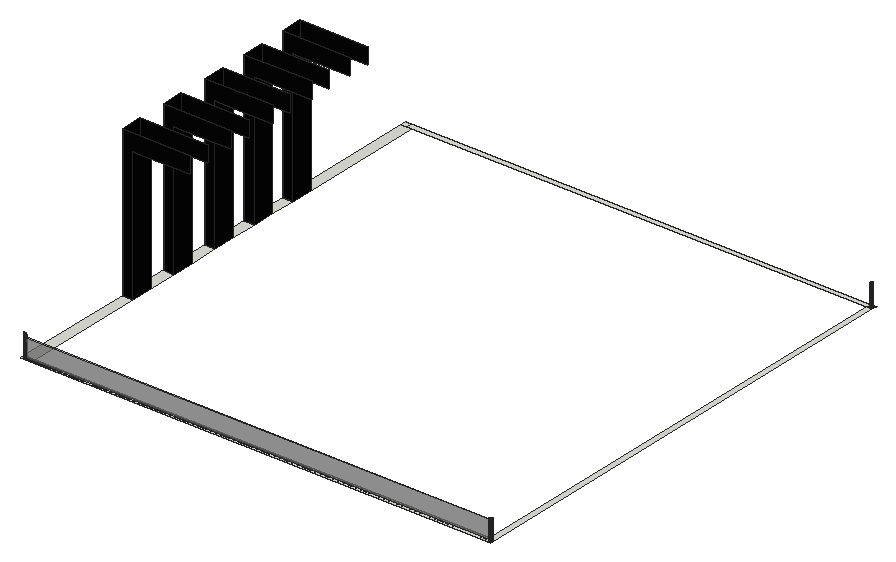
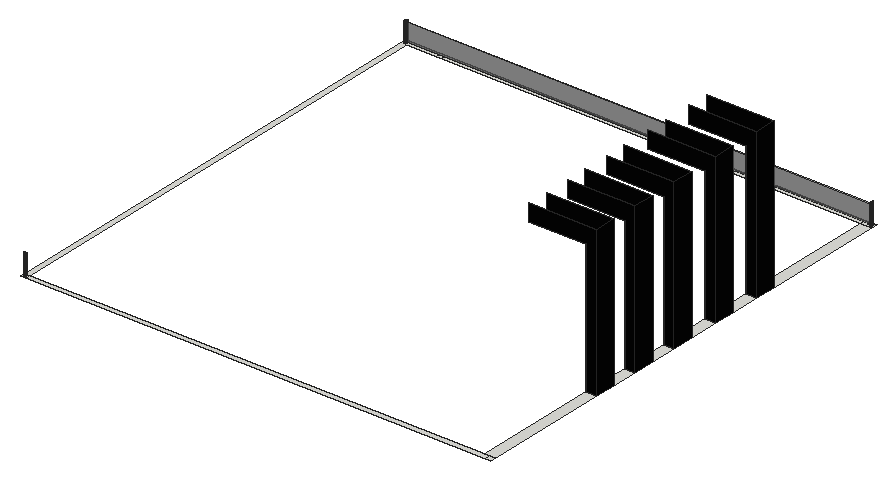
# SketchUp Ruby script. Lengths in inches.
U = 1.inch
M = Sketchup.active_model
def pt(a) = Geom::Point3d.new(a.map { |v| v * U })
def face(e, loops, mat)
  f = e.add_face(loops[0].map { |a| pt(a) })
  loops[1..].each { |l| e.add_face(l.map { |a| pt(a) }).erase! }
  f.material = f.back_material = mat if mat
  f
end
# faces: each face lists its corners as indices into pts; further lists are holes
def faces(e, pts, list, mat = nil) = list.each { |f| face(e, (f[0].is_a?(Array) ? f : [f]).map { |l| l.map { |i| pts[i] } }, mat) }
# xy, xz, yz: faces in a plane at the given z, y or x. An outline is a flat list of corners, or four numbers for a rectangle; further outlines are holes
def ring(l) = l.size == 4 ? [[l[0], l[1]], [l[2], l[1]], [l[2], l[3]], [l[0], l[3]]] : l.each_slice(2).to_a
def flat(e, list, mat, &to3) = list.each { |f| face(e, (f[0].is_a?(Array) ? f : [f]).map { |l| ring(l).map { |u, v| to3.(u, v) } }, mat) }
def xy(e, z, list, mat = nil) = flat(e, list, mat) { |x, y| [x, y, z] }
def xz(e, y, list, mat = nil) = flat(e, list, mat) { |x, z| [x, y, z] }
def yz(e, x, list, mat = nil) = flat(e, list, mat) { |y, z| [x, y, z] }
def lines(e, pts, list) = list.each { |a, b| e.add_line(pt(pts[a]), pt(pts[b])) }
# prism: a flat outline (further loops are holes) pulled along v
def prism(e, loops, v, mat = nil)
  f = face(e, loops, mat); d = Geom::Vector3d.new(v.map { |x| x * U })
  f.pushpull(f.normal.samedirection?(d) ? d.length : -d.length)
end
def box(e, o, s, mat = nil) = prism(e, [[o, [o[0] + s[0], o[1], o[2]], [o[0] + s[0], o[1] + s[1], o[2]], [o[0], o[1] + s[1], o[2]]]], [0, 0, s[2]], mat)
def at(x, y, z, deg = 0) = Geom::Transformation.translation(pt([x, y, z])) * Geom::Transformation.rotation(ORIGIN, Z_AXIS, deg.degrees)
def axes(o, x, y, z) = Geom::Transformation.new([*x, 0, *y, 0, *z, 0, *pt(o).to_a, 1])
def part(name) = M.definitions.add(name)
# library, detail: a bought-in or finely detailed component or shape, given as its bounding box
def library(name, o, s) = part(name).tap { |d| box(d.entities, o, s) }
def detail(e, o, s) = box(e.add_group.entities, o, s)
def put(e, d, t, mat = nil) = e.add_instance(d, t).tap { |i| i.material = mat if mat }
def group(e, t, mat = nil) = e.add_group.tap { |g| g.transformation = t; g.material = mat if mat }.entities
root = M.entities
M.materials.add("[0136_Charcoal]").color = [5, 5, 5]
M.materials.add("[0137_Black]").color = [0, 0, 0]
M.materials.add("[Translucent Glass Gray]").color = [128, 128, 128]
M.materials["[Translucent Glass Gray]"].alpha = 0.5
xy(root,1309.0625,[[0,72.375,12,72.375,12,75.58,8.99,75.58,8.99,78.17,8.98,78.0625,8.93,77.75,8.85,77.45,8.74,77.15,8.6,76.875,8.43,76.61,8.23,76.37,8.01,76.15,7.76,75.95,7.5,75.78,7.22,75.63,6.93,75.52,6.625,75.44,6.3125,75.39,6,75.375,5.6875,75.39,5.375,75.44,5.07,75.52,4.78,75.63,4.5,75.78,4.24,75.95,3.99,76.15,3.77,76.37,3.57,76.61,3.4,76.875,3.26,77.15,3.15,77.45,3.07,77.75,3.02,78.0625,3,78.375,3.02,78.6875,3.07,79,3.15,79.3,3.26,79.6,3.4,79.875,3.57,80.14,3.77,80.38,3.99,80.6,4.24,80.8,4.5,80.97,4.78,81.12,5.07,81.23,5.375,81.31,5.6875,81.36,6,81.375,6.3125,81.36,6.625,81.31,6.93,81.23,7.22,81.12,7.5,80.97,7.76,80.8,8.01,80.6,8.23,80.38,8.43,80.14,8.6,79.875,8.74,79.6,8.85,79.3,8.93,79,8.98,78.6875,8.99,78.58,12,78.58,12,84.375,0,84.375],[12,72.375,1086,72.375,1086,1170.375,1074,1170.375,1074,84.375,12,84.375,12,78.58,1077.01,78.58,1077.04,78.89,1077.11,79.2,1077.22,79.49,1077.35,79.78,1077.51,80.05,1077.7,80.3,1077.91,80.53,1078.15,80.74,1078.41,80.92,1078.68,81.07,1078.97,81.19,1079.27,81.28,1079.58,81.35,1079.89,81.37,1080.2,81.37,1080.52,81.33,1080.82,81.26,1081.12,81.16,1081.4,81.03,1081.67,80.86,1081.92,80.68,1082.15,80.46,1082.36,80.23,1082.54,79.97,1082.69,79.69,1082.82,79.41,1082.91,79.11,1082.97,78.8,1083,78.48,1082.99,78.17,1082.96,77.86,1082.89,77.55,1082.78,77.26,1082.65,76.97,1082.49,76.7,1082.3,76.45,1082.09,76.22,1081.85,76.01,1081.59,75.83,1081.32,75.68,1081.03,75.56,1080.73,75.47,1080.42,75.4,1080.11,75.38,1079.8,75.38,1079.48,75.42,1079.18,75.49,1078.88,75.59,1078.6,75.72,1078.33,75.89,1078.08,76.07,1077.85,76.29,1077.64,76.52,1077.46,76.78,1077.31,77.06,1077.18,77.34,1077.09,77.64,1077.03,77.95,1077.01,78.21,1077.01,75.58,12,75.58],[6,75.375,5.6875,75.39,5.375,75.44,5.07,75.52,4.78,75.63,4.5,75.78,4.24,75.95,3.99,76.15,3.77,76.37,3.57,76.61,3.4,76.875,3.26,77.15,3.15,77.45,3.07,77.75,3.02,78.0625,3,78.375,3.02,78.6875,3.07,79,3.15,79.3,3.26,79.6,3.4,79.875,3.57,80.14,3.77,80.38,3.99,80.6,4.24,80.8,4.5,80.97,4.78,81.12,5.07,81.23,5.375,81.31,5.6875,81.36,6,81.375,6.3125,81.36,6.625,81.31,6.93,81.23,7.22,81.12,7.5,80.97,7.76,80.8,8.01,80.6,8.23,80.38,8.43,80.14,8.6,79.875,8.74,79.6,8.85,79.3,8.93,79,8.98,78.6875,8.99,78.58,8.99,78.17,8.98,78.0625,8.93,77.75,8.85,77.45,8.74,77.15,8.6,76.875,8.43,76.61,8.23,76.37,8.01,76.15,7.76,75.95,7.5,75.78,7.22,75.63,6.93,75.52,6.625,75.44,6.3125,75.39],[1079.8,75.38,1079.48,75.42,1079.18,75.49,1078.88,75.59,1078.6,75.72,1078.33,75.89,1078.08,76.07,1077.85,76.29,1077.64,76.52,1077.46,76.78,1077.31,77.06,1077.18,77.34,1077.09,77.64,1077.03,77.95,1077.01,78.21,1077.01,78.58,1077.04,78.89,1077.11,79.2,1077.22,79.49,1077.35,79.78,1077.51,80.05,1077.7,80.3,1077.91,80.53,1078.15,80.74,1078.41,80.92,1078.68,81.07,1078.97,81.19,1079.27,81.28,1079.58,81.35,1079.89,81.37,1080.2,81.37,1080.52,81.33,1080.82,81.26,1081.12,81.16,1081.4,81.03,1081.67,80.86,1081.92,80.68,1082.15,80.46,1082.36,80.23,1082.54,79.97,1082.69,79.69,1082.82,79.41,1082.91,79.11,1082.97,78.8,1083,78.48,1082.99,78.17,1082.96,77.86,1082.89,77.55,1082.78,77.26,1082.65,76.97,1082.49,76.7,1082.3,76.45,1082.09,76.22,1081.85,76.01,1081.59,75.83,1081.32,75.68,1081.03,75.56,1080.73,75.47,1080.42,75.4,1080.11,75.38],[8.99,75.58,8.99,78.17,9,78.375,8.99,78.58,12,78.58,12,75.58],
  [12,75.58,12,78.58,1077.01,78.58,1077,78.27,1077.01,78.21,1077.01,75.58],[8.99,78.17,8.99,78.58,9,78.375],[1077.01,78.21,1077,78.27,1077.01,78.58],[0,84.375,24.25,366.56],[0,366.56,24.25,417.12],
  [0,417.12,24.25,484.62],[0,484.62,24.25,535.18],[0,535.18,24.25,604.12],[0,604.12,24.25,654.68],[0,654.68,24.25,717.12],
  [0,717.12,24.25,767.68],[0,767.68,24.25,827.68],[0,827.68,24.25,878.24],[0,878.24,24.25,1170.375],[0,1170.375,12,1182.375],
  [12,1170.375,1074,1182.375],[[1074,1170.375,1086,1182.375],[1079.86,1173.38,1079.55,1173.41,1079.24,1173.47,1078.94,1173.57,1078.65,1173.69,1078.38,1173.85,1078.125,1174.03,1077.89,1174.24,1077.68,1174.47,1077.49,1174.73,1077.34,1175,1077.21,1175.28,1077.11,1175.58,1077.04,1175.89,1077.01,1176.2,1077,1176.51,1077.03,1176.83,1077.1,1177.13,1077.19,1177.43,1077.32,1177.72,1077.47,1177.99,1077.66,1178.25,1077.87,1178.48,1078.1,1178.69,1078.35,1178.88,1078.62,1179.04,1078.91,1179.17,1079.21,1179.27,1079.51,1179.34,1079.82,1179.37,1080.14,1179.37,1080.45,1179.34,1080.76,1179.28,1081.06,1179.18,1081.35,1179.06,1081.62,1178.9,1081.875,1178.72,1082.11,1178.51,1082.32,1178.28,1082.51,1178.02,1082.66,1177.75,1082.79,1177.47,1082.89,1177.17,1082.96,1176.86,1082.99,1176.55,1083,1176.24,1082.97,1175.92,1082.9,1175.62,1082.81,1175.32,1082.68,1175.03,1082.53,1174.76,1082.34,1174.5,1082.13,1174.27,1081.9,1174.06,1081.65,1173.87,1081.38,1173.71,1081.09,1173.58,1080.79,1173.48,1080.49,1173.41,1080.18,1173.38]],[1079.86,1173.38,1079.55,1173.41,1079.24,1173.47,1078.94,1173.57,1078.65,1173.69,1078.38,1173.85,1078.125,1174.03,1077.89,1174.24,1077.68,1174.47,1077.49,1174.73,1077.34,1175,1077.21,1175.28,1077.11,1175.58,1077.04,1175.89,1077.01,1176.2,1077,1176.51,1077.03,1176.83,1077.1,1177.13,1077.19,1177.43,1077.32,1177.72,1077.47,1177.99,1077.66,1178.25,1077.87,1178.48,1078.1,1178.69,1078.35,1178.88,1078.62,1179.04,1078.91,1179.17,1079.21,1179.27,1079.51,1179.34,1079.82,1179.37,1080.14,1179.37,1080.45,1179.34,1080.76,1179.28,1081.06,1179.18,1081.35,1179.06,1081.62,1178.9,1081.875,1178.72,1082.11,1178.51,1082.32,1178.28,1082.51,1178.02,1082.66,1177.75,1082.79,1177.47,1082.89,1177.17,1082.96,1176.86,1082.99,1176.55,1083,1176.24,1082.97,1175.92,1082.9,1175.62,1082.81,1175.32,1082.68,1175.03,1082.53,1174.76,1082.34,1174.5,1082.13,1174.27,1081.9,1174.06,1081.65,1173.87,1081.38,1173.71,1081.09,1173.58,1080.79,1173.48,1080.49,1173.41,1080.18,1173.38]])
xz(root,75.38,[[1079.8,1309.0625,1080.11,1354.0625]],"[0137_Black]")
xz(root,75.58,[[8.99,1309.0625,1077.01,1352.375]],"[Translucent Glass Gray]")
xz(root,78.58,[[8.99,1309.0625,1077.01,1352.375]],"[Translucent Glass Gray]")
xz(root,81.37,[[1079.89,1309.0625,1080.2,1354.0625]],"[0137_Black]")
xz(root,366.56,[[0,1309.0625,24.25,1309.0625,24.25,1614.61,156,1614.61,156,1652.92,0,1652.92]],"[0136_Charcoal]")
xz(root,417.12,[[0,1309.0625,0,1652.92,156,1652.92,156,1614.61,24.25,1614.61,24.25,1309.0625]],"[0136_Charcoal]")
xz(root,484.62,[[0,1309.0625,24.25,1309.0625,24.25,1614.61,156,1614.61,156,1652.92,0,1652.92]],"[0136_Charcoal]")
xz(root,535.18,[[0,1309.0625,0,1652.92,156,1652.92,156,1614.61,24.25,1614.61,24.25,1309.0625]],"[0136_Charcoal]")
xz(root,604.12,[[0,1309.0625,24.25,1309.0625,24.25,1614.61,156,1614.61,156,1652.92,0,1652.92]],"[0136_Charcoal]")
xz(root,654.68,[[0,1309.0625,0,1652.92,156,1652.92,156,1614.61,24.25,1614.61,24.25,1309.0625]],"[0136_Charcoal]")
xz(root,717.12,[[0,1309.0625,24.25,1309.0625,24.25,1614.61,156,1614.61,156,1652.92,0,1652.92]],"[0136_Charcoal]")
xz(root,767.68,[[0,1309.0625,0,1652.92,156,1652.92,156,1614.61,24.25,1614.61,24.25,1309.0625]],"[0136_Charcoal]")
xz(root,827.68,[[0,1309.0625,24.25,1309.0625,24.25,1614.61,156,1614.61,156,1652.92,0,1652.92]],"[0136_Charcoal]")
xz(root,878.24,[[0,1309.0625,0,1652.92,156,1652.92,156,1614.61,24.25,1614.61,24.25,1309.0625]],"[0136_Charcoal]")
xz(root,1173.38,[[1079.86,1309.0625,1080.18,1354.07]],"[0137_Black]")
xz(root,1179.37,[[1079.82,1309.0625,1080.14,1360.06]],"[0137_Black]")
yz(root,0,[[366.56,1309.0625,417.12,1652.92],[484.62,1309.0625,535.18,1652.92],[604.12,1309.0625,654.68,1652.92],[717.12,1309.0625,767.68,1652.92],[827.68,1309.0625,878.24,1652.92]],"[0136_Charcoal]")
yz(root,8.99,[[75.58,1309.0625,78.58,1352.375]])
yz(root,24.25,[[366.56,1309.0625,417.12,1614.61],[484.62,1309.0625,535.18,1614.61],[604.12,1309.0625,654.68,1614.61],[717.12,1309.0625,767.68,1614.61],[827.68,1309.0625,878.24,1614.61]],"[0136_Charcoal]")
yz(root,1077.01,[[75.58,1309.0625,78.58,1352.375]])
p = [[5.07,75.52,1309.0625],[5.375,75.44,1309.0625],[5.375,75.44,1357.6875],[5.07,75.52,1357.99],[5.6875,75.39,1309.0625],[5.6875,75.39,1357.375],
  [6,75.375,1309.0625],[6,75.375,1357.0625],[6.3125,75.39,1309.0625],[6.3125,75.39,1356.75],[6.625,75.44,1309.0625],[6.625,75.44,1356.4375],
  [6.93,75.52,1309.0625],[6.93,75.52,1356.14],[1079.18,75.49,1309.0625],[1079.48,75.42,1309.0625],[1079.48,75.42,1354.0625],[1079.18,75.49,1354.0625],
  [1079.8,75.38,1309.0625],[1079.8,75.38,1354.0625],[1080.11,75.38,1309.0625],[1080.42,75.4,1309.0625],[1080.42,75.4,1354.0625],[1080.11,75.38,1354.0625],
  [1080.73,75.47,1309.0625],[1080.73,75.47,1354.0625],[4.78,75.63,1309.0625],[4.78,75.63,1358.28],[7.22,75.63,1309.0625],[7.22,75.63,1355.84],
  [1078.88,75.59,1309.0625],[1078.88,75.59,1354.0625],[1081.03,75.56,1309.0625],[1081.03,75.56,1354.0625],[4.5,75.78,1309.0625],[4.5,75.78,1358.5625],
  [7.5,75.78,1309.0625],[7.5,75.78,1355.5625],[1078.6,75.72,1309.0625],[1078.6,75.72,1354.0625],[1081.32,75.68,1309.0625],[1081.32,75.68,1354.0625],
  [1078.33,75.89,1309.0625],[1078.33,75.89,1354.0625],[1081.59,75.83,1309.0625],[1081.59,75.83,1354.0625],[4.24,75.95,1309.0625],[4.24,75.95,1358.83],
  [7.76,75.95,1309.0625],[7.76,75.95,1355.3],[1081.85,76.01,1309.0625],[1081.85,76.01,1354.0625],[3.99,76.15,1309.0625],[3.99,76.15,1359.07],
  [8.01,76.15,1309.0625],[8.01,76.15,1355.06],[1078.08,76.07,1309.0625],[1078.08,76.07,1354.0625],[1082.09,76.22,1309.0625],[1082.09,76.22,1354.0625],
  [3.77,76.37,1309.0625],[3.77,76.37,1359.29],[8.23,76.37,1309.0625],[8.23,76.37,1354.83],[1077.85,76.29,1309.0625],[1077.85,76.29,1354.0625],
  [1082.3,76.45,1309.0625],[1082.3,76.45,1354.0625],[1077.64,76.52,1309.0625],[1077.64,76.52,1354.0625],[3.57,76.61,1309.0625],[3.57,76.61,1359.49],
  [8.43,76.61,1309.0625],[8.43,76.61,1354.64],[1077.46,76.78,1309.0625],[1077.46,76.78,1354.0625],[1082.49,76.7,1309.0625],[1082.49,76.7,1354.0625],
  [3.4,76.875,1309.0625],[3.4,76.875,1359.66],[8.6,76.875,1309.0625],[8.6,76.875,1354.46],[1082.65,76.97,1309.0625],[1082.65,76.97,1354.0625],
  [1077.31,77.06,1309.0625],[1077.31,77.06,1354.0625],[3.26,77.15,1309.0625],[3.26,77.15,1359.8],[8.74,77.15,1309.0625],[8.74,77.15,1354.32],
  [1082.78,77.26,1309.0625],[1082.78,77.26,1354.0625],[1077.18,77.34,1309.0625],[1077.18,77.34,1354.0625],[3.15,77.45,1309.0625],[3.15,77.45,1359.92],
  [8.85,77.45,1309.0625],[8.85,77.45,1354.21],[1077.09,77.64,1309.0625],[1077.09,77.64,1354.0625],[1082.89,77.55,1309.0625],[1082.89,77.55,1354.0625],
  [3.07,77.75,1309.0625],[3.07,77.75,1360],[8.93,77.75,1309.0625],[8.93,77.75,1354.13],[1077.03,77.95,1309.0625],[1077.03,77.95,1354.0625],
  [1082.96,77.86,1309.0625],[1082.96,77.86,1354.0625],[3.02,78.0625,1309.0625],[3.02,78.0625,1360.05],[8.98,78.0625,1309.0625],[8.98,78.0625,1354.08],
  [1082.99,78.17,1309.0625],[1082.99,78.17,1354.0625],[1077,78.27,1309.0625],[1077.01,78.21,1309.0625],[1077,78.27,1354.0625],[3,78.375,1309.0625],
  [3,78.375,1360.0625],[8.99,78.17,1309.0625],[9,78.375,1309.0625],[9,78.375,1354.0625],[1083,78.48,1309.0625],[1083,78.48,1354.0625],
  [1077.01,78.58,1309.0625],[1077,78.375,1354.0625],[1077.01,78.58,1354.0625],[1077.01,78.58,1352.375],[3.02,78.6875,1309.0625],[3.02,78.6875,1360.05],
  [8.99,78.58,1309.0625],[8.98,78.6875,1309.0625],[8.98,78.6875,1354.08],[1082.97,78.8,1309.0625],[1082.97,78.8,1354.0625],[1077.04,78.89,1309.0625],
  [1077.04,78.89,1354.0625],[3.07,79,1309.0625],[3.07,79,1360],[8.93,79,1309.0625],[8.93,79,1354.13],[1082.91,79.11,1309.0625],
  [1082.91,79.11,1354.0625],[1077.11,79.2,1309.0625],[1077.11,79.2,1354.0625],[3.15,79.3,1309.0625],[3.15,79.3,1359.92],[8.85,79.3,1309.0625],
  [8.85,79.3,1354.21],[1082.82,79.41,1309.0625],[1082.82,79.41,1354.0625],[1077.22,79.49,1309.0625],[1077.22,79.49,1354.0625],[3.26,79.6,1309.0625],
  [3.26,79.6,1359.8],[8.74,79.6,1309.0625],[8.74,79.6,1354.32],[1082.69,79.69,1309.0625],[1082.69,79.69,1354.0625],[1077.35,79.78,1309.0625],
  [1077.35,79.78,1354.0625],[3.4,79.875,1309.0625],[3.4,79.875,1359.66],[8.6,79.875,1309.0625],[8.6,79.875,1354.46],[1082.54,79.97,1309.0625],
  [1082.54,79.97,1354.0625],[1077.51,80.05,1309.0625],[1077.51,80.05,1354.0625],[3.57,80.14,1309.0625],[3.57,80.14,1359.49],[8.43,80.14,1309.0625],
  [8.43,80.14,1354.64],[1077.7,80.3,1309.0625],[1077.7,80.3,1354.0625],[1082.36,80.23,1309.0625],[1082.36,80.23,1354.0625],[3.77,80.38,1309.0625],
  [3.77,80.38,1359.29],[8.23,80.38,1309.0625],[8.23,80.38,1354.83],[1082.15,80.46,1309.0625],[1082.15,80.46,1354.0625],[1077.91,80.53,1309.0625],
  [1077.91,80.53,1354.0625],[3.99,80.6,1309.0625],[3.99,80.6,1359.07],[8.01,80.6,1309.0625],[8.01,80.6,1355.06],[1078.15,80.74,1309.0625],
  [1078.15,80.74,1354.0625],[1081.92,80.68,1309.0625],[1081.92,80.68,1354.0625],[4.24,80.8,1309.0625],[4.24,80.8,1358.83],[7.76,80.8,1309.0625],
  [7.76,80.8,1355.3],[1078.41,80.92,1309.0625],[1078.41,80.92,1354.0625],[1081.67,80.86,1309.0625],[1081.67,80.86,1354.0625],[4.5,80.97,1309.0625],
  [4.5,80.97,1358.5625],[7.5,80.97,1309.0625],[7.5,80.97,1355.5625],[1078.68,81.07,1309.0625],[1078.68,81.07,1354.0625],[1081.4,81.03,1309.0625],
  [1081.4,81.03,1354.0625],[4.78,81.12,1309.0625],[4.78,81.12,1358.28],[7.22,81.12,1309.0625],[7.22,81.12,1355.84],[1081.12,81.16,1309.0625],
  [1081.12,81.16,1354.0625],[5.07,81.23,1309.0625],[5.07,81.23,1357.99],[6.93,81.23,1309.0625],[6.93,81.23,1356.14],[1078.97,81.19,1309.0625],
  [1078.97,81.19,1354.0625],[5.375,81.31,1309.0625],[5.375,81.31,1357.6875],[6.625,81.31,1309.0625],[6.625,81.31,1356.4375],[1079.27,81.28,1309.0625],
  [1079.27,81.28,1354.0625],[1080.82,81.26,1309.0625],[1080.82,81.26,1354.0625],[5.6875,81.36,1309.0625],[5.6875,81.36,1357.375],[6.3125,81.36,1309.0625],
  [6.3125,81.36,1356.75],[1079.58,81.35,1309.0625],[1079.58,81.35,1354.0625],[1079.89,81.37,1309.0625],[1079.89,81.37,1354.0625],[1080.52,81.33,1309.0625],
  [1080.2,81.37,1309.0625],[1080.2,81.37,1354.0625],[1080.52,81.33,1354.0625],[6,81.375,1309.0625],[6,81.375,1357.0625],[6,81.375,1354.0625],
  [1079.24,1173.47,1309.0625],[1079.55,1173.41,1309.0625],[1079.55,1173.41,1354.1],[1079.24,1173.47,1354.16],[1079.86,1173.38,1309.0625],[1079.86,1173.38,1354.07],
  [1080.18,1173.38,1309.0625],[1080.49,1173.41,1309.0625],[1080.49,1173.41,1354.1],[1080.18,1173.38,1354.07],[1080.79,1173.48,1309.0625],[1080.79,1173.48,1354.17],
  [1078.94,1173.57,1309.0625],[1078.94,1173.57,1354.26],[1081.09,1173.58,1309.0625],[1081.09,1173.58,1354.27],[1078.65,1173.69,1309.0625],[1078.65,1173.69,1354.38],
  [1081.38,1173.71,1309.0625],[1081.38,1173.71,1354.4],[1078.38,1173.85,1309.0625],[1078.38,1173.85,1354.54],[1081.65,1173.87,1309.0625],[1081.65,1173.87,1354.56],
  [1078.125,1174.03,1309.0625],[1078.125,1174.03,1354.72],[1081.9,1174.06,1309.0625],[1081.9,1174.06,1354.74],[1077.89,1174.24,1309.0625],[1077.89,1174.24,1354.93],
  [1082.13,1174.27,1309.0625],[1082.13,1174.27,1354.95],[1077.68,1174.47,1309.0625],[1077.68,1174.47,1355.16],[1082.34,1174.5,1309.0625],[1082.34,1174.5,1355.1875],
  [1077.49,1174.73,1309.0625],[1077.49,1174.73,1355.41],[1082.53,1174.76,1309.0625],[1082.53,1174.76,1355.44],[1077.34,1175,1309.0625],[1077.34,1175,1355.68],
  [1082.68,1175.03,1309.0625],[1082.68,1175.03,1355.72],[1077.21,1175.28,1309.0625],[1077.21,1175.28,1355.97],[1082.81,1175.32,1309.0625],[1082.81,1175.32,1356],
  [1077.11,1175.58,1309.0625],[1077.11,1175.58,1356.27],[1082.9,1175.62,1309.0625],[1082.9,1175.62,1356.3],[1077.04,1175.89,1309.0625],[1077.04,1175.89,1356.57],
  [1082.97,1175.92,1309.0625],[1082.97,1175.92,1356.61],[1077.01,1176.2,1309.0625],[1077.01,1176.2,1356.89],[1077.01,1176.2,1354.09],[1083,1176.24,1309.0625],
  [1083,1176.24,1356.92],[1077,1176.51,1354.07],[1077,1176.51,1309.0625],[1082.99,1176.55,1309.0625],[1082.99,1176.55,1357.24],[1077.03,1176.83,1309.0625],
  [1077,1176.51,1357.2],[1077.03,1176.83,1357.51],[1082.96,1176.86,1309.0625],[1082.96,1176.86,1357.55],[1077.1,1177.13,1309.0625],[1077.1,1177.13,1357.82],
  [1082.89,1177.17,1309.0625],[1082.89,1177.17,1357.86],[1077.19,1177.43,1309.0625],[1077.19,1177.43,1358.12],[1082.79,1177.47,1309.0625],[1082.79,1177.47,1358.15],
  [1077.32,1177.72,1309.0625],[1077.32,1177.72,1358.41],[1082.66,1177.75,1309.0625],[1082.66,1177.75,1358.44],[1077.47,1177.99,1309.0625],[1077.47,1177.99,1358.68],
  [1082.51,1178.02,1309.0625],[1082.51,1178.02,1358.71],[1077.66,1178.25,1309.0625],[1077.66,1178.25,1358.9375],[1082.32,1178.28,1309.0625],[1082.32,1178.28,1358.96],
  [1077.87,1178.48,1309.0625],[1077.87,1178.48,1359.17],[1082.11,1178.51,1309.0625],[1082.11,1178.51,1359.2],[1078.1,1178.69,1309.0625],[1078.1,1178.69,1359.38],
  [1081.875,1178.72,1309.0625],[1081.875,1178.72,1359.41],[1078.35,1178.88,1309.0625],[1078.35,1178.88,1359.57],[1081.62,1178.9,1309.0625],[1081.62,1178.9,1359.59],
  [1078.62,1179.04,1309.0625],[1078.62,1179.04,1359.73],[1081.35,1179.06,1309.0625],[1081.35,1179.06,1359.74],[1078.91,1179.17,1309.0625],[1078.91,1179.17,1359.86],
  [1081.06,1179.18,1309.0625],[1081.06,1179.18,1359.87],[1079.21,1179.27,1309.0625],[1079.21,1179.27,1359.96],[1080.76,1179.28,1309.0625],[1080.76,1179.28,1359.96],
  [1079.51,1179.34,1309.0625],[1079.51,1179.34,1360.02],[1079.82,1179.37,1309.0625],[1079.82,1179.37,1360.06],[1080.45,1179.34,1309.0625],[1080.14,1179.37,1309.0625],
  [1080.14,1179.37,1360.06],[1080.45,1179.34,1360.03],[1080,78.375,1309.0625],[1080,78.375,1354.0625],[6,78.375,1309.0625],[6,78.375,1357.0625],
  [1080,1176.375,1309.0625],[1080,1176.375,1357.0625]]
faces(root,p,[[0,1,2,3],[1,4,5,2],[4,6,7,5],[6,8,9,7],[8,10,11,9],[10,12,13,11],[14,15,16,17],[15,18,19,16],
  [20,21,22,23],[21,24,25,22],[26,0,3,27],[12,28,29,13],[30,14,17,31],[24,32,33,25],[34,26,27,35],[28,36,37,29],
  [38,30,31,39],[32,40,41,33],[42,38,39,43],[40,44,45,41],[46,34,35,47],[36,48,49,37],[44,50,51,45],[52,46,47,53],
  [48,54,55,49],[56,42,43,57],[50,58,59,51],[60,52,53,61],[54,62,63,55],[64,56,57,65],[58,66,67,59],[68,64,65,69],
  [70,60,61,71],[62,72,73,63],[74,68,69,75],[66,76,77,67],[72,80,81,73],[76,82,83,77],[84,74,75,85],[80,88,89,81],
  [82,90,91,83],[92,84,85,93],[88,96,97,89],[98,92,93,99],[90,100,101,91],[96,104,105,97],[106,98,99,107],[100,108,109,101],
  [108,114,115,109],[116,117,106,107,118],[114,124,125,115],[126,116,118,127,128,129],[124,135,136,125],[137,126,129,128,138],[135,143,144,136],[145,137,138,146],
  [143,151,152,144],[153,145,146,154],[151,159,160,152],[161,153,154,162],[159,167,168,160],[169,161,162,170],[175,169,170,176],[167,177,178,168],
  [177,183,184,178],[185,175,176,186],[191,185,186,192],[183,193,194,184],[199,191,192,200],[193,201,202,194],[207,199,200,208],[201,209,210,202],
  [209,215,216,210],[221,207,208,222],[227,221,222,228],[215,229,230,216],[235,227,228,236],[237,235,236,238],[239,240,241,242],[229,239,242,230],
  [246,247,248,249],[247,250,251,248],[252,253,254,255],[253,256,257,254],[258,246,249,259],[256,260,261,257],[262,258,259,263],[260,264,265,261],
  [266,262,263,267],[264,268,269,265],[270,266,267,271],[268,272,273,269],[274,270,271,275],[272,276,277,273],[278,274,275,279],[276,280,281,277],
  [282,278,279,283],[280,284,285,281],[286,282,283,287],[284,288,289,285],[290,286,287,291],[288,292,293,289],[294,290,291,295],[292,296,297,293],
  [298,294,295,299],[296,300,301,297],[302,298,299,303,304],[300,305,306,301],[302,304,307,308],[305,309,310,306],[311,308,307,312,313],[309,314,315,310],
  [316,311,313,317],[314,318,319,315],[320,316,317,321],[318,322,323,319],[324,320,321,325],[322,326,327,323],[328,324,325,329],[326,330,331,327],
  [332,328,329,333],[330,334,335,331],[336,332,333,337],[334,338,339,335],[340,336,337,341],[338,342,343,339],[344,340,341,345],[342,346,347,343],
  [348,344,345,349],[346,350,351,347],[352,348,349,353],[350,354,355,351],[356,352,353,357],[354,358,359,355],[360,356,357,361],[362,360,361,363],
  [364,365,366,367],[358,364,367,359]],"[0137_Black]")
faces(root,p,[[78,70,71,79],[86,78,79,87],[94,86,87,95],[102,94,95,103],[110,102,103,111],[104,112,113,105],[119,110,111,120],[112,121,122,123,113],
  [130,119,120,131],[122,132,133,134,123],[139,130,131,140],[133,141,142,134],[147,139,140,148],[141,149,150,142],[155,147,148,156],[149,157,158,150],
  [163,155,156,164],[157,165,166,158],[171,163,164,172],[165,173,174,166],[179,171,172,180],[173,181,182,174],[187,179,180,188],[181,189,190,182],
  [195,187,188,196],[189,197,198,190],[203,195,196,204],[197,205,206,198],[211,203,204,212],[205,213,214,206],[217,211,212,218],[213,219,220,214],
  [223,217,218,224],[219,225,226,220],[231,223,224,232],[225,233,234,226],[243,231,232,244,245],[233,243,245,244,234]])
lines(root,p,[[368,369],[370,371],[372,373]])
